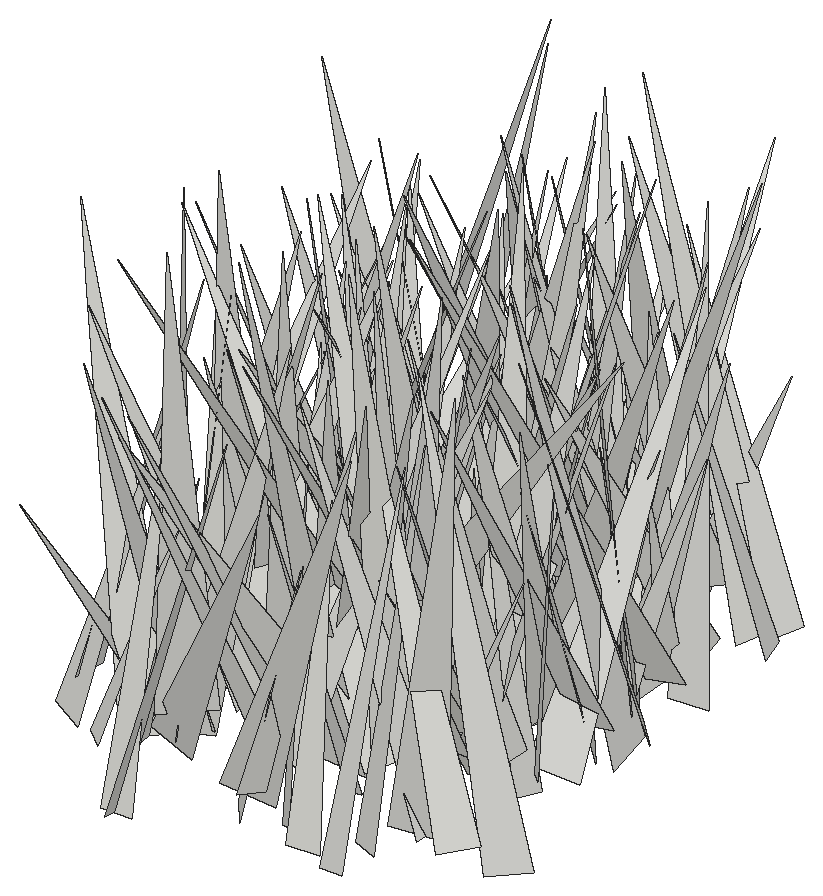
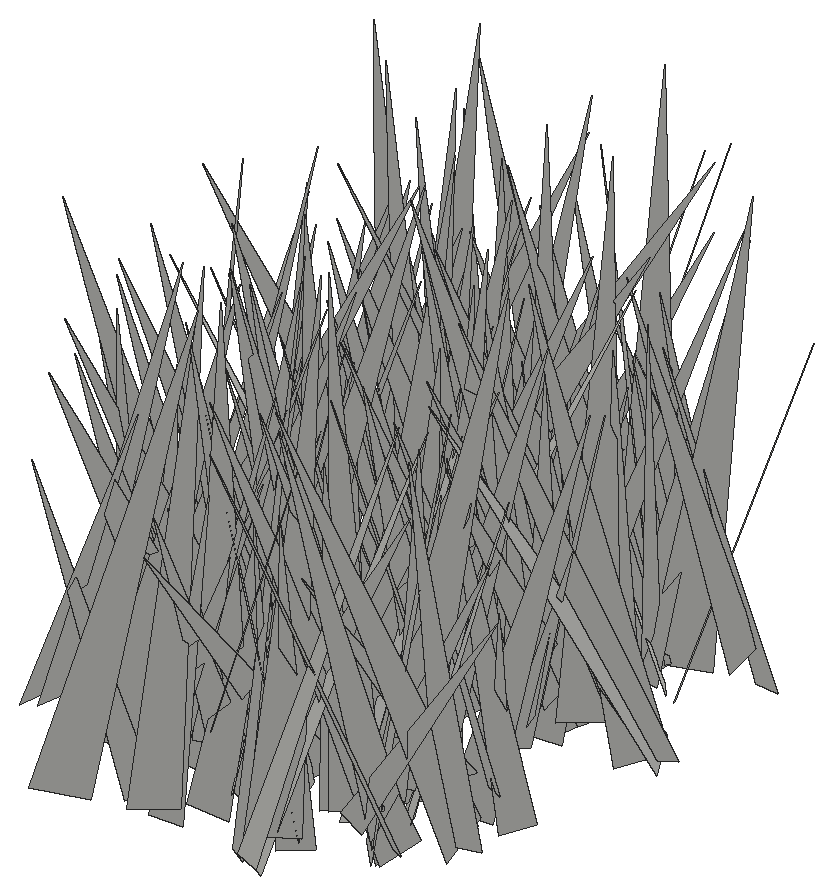
# SketchUp Ruby script. Lengths in inches.
U = 1.inch
M = Sketchup.active_model
def pt(a) = Geom::Point3d.new(a.map { |v| v * U })
def face(e, loops, mat)
  f = e.add_face(loops[0].map { |a| pt(a) })
  loops[1..].each { |l| e.add_face(l.map { |a| pt(a) }).erase! }
  f.material = f.back_material = mat if mat
  f
end
# faces: each face lists its corners as indices into pts; further lists are holes
def faces(e, pts, list, mat = nil) = list.each { |f| face(e, (f[0].is_a?(Array) ? f : [f]).map { |l| l.map { |i| pts[i] } }, mat) }
# xy, xz, yz: faces in a plane at the given z, y or x. An outline is a flat list of corners, or four numbers for a rectangle; further outlines are holes
def ring(l) = l.size == 4 ? [[l[0], l[1]], [l[2], l[1]], [l[2], l[3]], [l[0], l[3]]] : l.each_slice(2).to_a
def flat(e, list, mat, &to3) = list.each { |f| face(e, (f[0].is_a?(Array) ? f : [f]).map { |l| ring(l).map { |u, v| to3.(u, v) } }, mat) }
def xy(e, z, list, mat = nil) = flat(e, list, mat) { |x, y| [x, y, z] }
def xz(e, y, list, mat = nil) = flat(e, list, mat) { |x, z| [x, y, z] }
def yz(e, x, list, mat = nil) = flat(e, list, mat) { |y, z| [x, y, z] }
def lines(e, pts, list) = list.each { |a, b| e.add_line(pt(pts[a]), pt(pts[b])) }
# prism: a flat outline (further loops are holes) pulled along v
def prism(e, loops, v, mat = nil)
  f = face(e, loops, mat); d = Geom::Vector3d.new(v.map { |x| x * U })
  f.pushpull(f.normal.samedirection?(d) ? d.length : -d.length)
end
def box(e, o, s, mat = nil) = prism(e, [[o, [o[0] + s[0], o[1], o[2]], [o[0] + s[0], o[1] + s[1], o[2]], [o[0], o[1] + s[1], o[2]]]], [0, 0, s[2]], mat)
def at(x, y, z, deg = 0) = Geom::Transformation.translation(pt([x, y, z])) * Geom::Transformation.rotation(ORIGIN, Z_AXIS, deg.degrees)
def axes(o, x, y, z) = Geom::Transformation.new([*x, 0, *y, 0, *z, 0, *pt(o).to_a, 1])
def part(name) = M.definitions.add(name)
# library, detail: a bought-in or finely detailed component or shape, given as its bounding box
def library(name, o, s) = part(name).tap { |d| box(d.entities, o, s) }
def detail(e, o, s) = box(e.add_group.entities, o, s)
def put(e, d, t, mat = nil) = e.add_instance(d, t).tap { |i| i.material = mat if mat }
def group(e, t, mat = nil) = e.add_group.tap { |g| g.transformation = t; g.material = mat if mat }.entities
root = M.entities
c1 = part("fur_instance\#9")
p = [[0.8125,0,1.79],[0.67,-0.02,1.48],[0,-0.11,0],[0,0.11,0]]
faces(c1.entities,p,[[0,1,2,3]])
put(root,c1,axes([141.56,90.83,-28.22],[2.97269,-7.01093,0.81561],[-6.80259,-2.60982,2.35986],[1.88234,1.64042,7.24024]))
put(root,c1,axes([139.31,87.79,-28.22],[5.0446,1.96996,1.21492],[1.59207,-5.06819,1.60732],[-1.6799,1.1124,5.17158]))
put(root,c1,axes([139.39,87.84,-28.22],[0.92539,5.82013,0.73982],[5.78512,-1.02986,0.86568],[-0.97656,-0.58571,5.82931]))
put(root,c1,axes([147.1875,87.4,-27.1],[1.91748,5.33638,0.31642],[5.10909,-1.9283,1.55969],[-1.57297,0.24194,5.4517]))
put(root,c1,axes([141.93,89.99,-28.22],[3.37975,2.64749,1.02841],[2.82915,-3.2791,-0.85611],[-0.25046,-1.31446,4.20701]))
put(root,c1,axes([138.12,91.8125,-28.22],[0.97454,-6.53217,0.4424],[-5.83998,-0.6651,3.04417],[2.95966,0.83851,5.86106]))
put(root,c1,axes([140.95,92.76,-28.22],[-5.93761,-4.29126,0.84113],[-3.95201,5.87307,2.0655],[1.8719,-1.21235,7.02879]))
put(root,c1,axes([144.63,89.375,-28.22],[-0.41482,4.98169,1.32883],[5.15587,0.40286,0.09923],[0.00793,-1.33251,4.99795]))
put(root,c1,axes([137.57,89.15,-27.1],[2.54826,3.20038,0.28055],[3.20908,-2.5526,-0.02947],[-0.15164,-0.23787,4.09087]))
put(root,c1,axes([136.37,93.4,-28.22],[-4.06772,-3.26977,0.32403],[-2.78571,3.7053,2.41936],[1.74246,-1.70943,4.62433]))
put(root,c1,axes([138.67,91.83,-27.1],[5.1556,-5.75467,2.21602],[-5.90961,-5.43588,-0.36737],[-1.76168,1.39363,7.71761]))
put(root,c1,axes([140.66,94.3,-28.22],[-5.78164,-4.6449,0.78576],[-4.06196,5.54542,2.89287],[2.386,-1.8147,6.82889]))
put(root,c1,axes([144.97,91.2,-27.1],[0.7235,3.49331,2.20248],[3.65755,-1.58024,1.30491],[-1.91742,-1.69623,3.32022]))
put(root,c1,axes([142.81,89.42,-27.1],[5.29795,0.17393,1.896],[-0.4687,-5.31448,1.7972],[-1.84537,1.84915,4.98684]))
put(root,c1,axes([141.83,93.98,-27.1],[2.44843,-5.51273,0.60157],[-4.8536,-2.44839,-2.68234],[-2.6823,-0.60174,5.40279]))
put(root,c1,axes([146.49,92.05,-28.22],[2.7668,-7.06079,2.0724],[-7.35623,-2.5972,0.97226],[0.18857,2.28135,7.52095]))
put(root,c1,axes([138.97,91.04,-27.1],[5.52113,3.74347,2.2115],[4.00437,-5.77059,-0.2291],[-1.6939,-1.44011,6.66663]))
put(root,c1,axes([138.02,92.97,-28.22],[-0.27695,-6.43694,1.01641],[-6.49492,0.18954,-0.56932],[-0.53231,1.03627,6.4177]))
put(root,c1,axes([137.47,91.25,-28.22],[4.33952,0.70183,1.00017],[0.70812,-4.45199,0.05164],[-0.99573,-0.10739,4.3956]))
put(root,c1,axes([134.91,91.28,-28.22],[2.00403,4.77087,1.2081],[4.88814,-1.77806,-1.08691],[0.57161,-1.52123,5.05925]))
put(root,c1,axes([149.17,90.4375,-27.1],[-2.13966,5.92839,0.3544],[5.56639,1.87053,2.31645],[-2.07043,-1.09766,5.86157]))
put(root,c1,axes([145.89,90.5,-28.22],[2.59525,5.12132,1.23508],[5.09738,-2.78884,0.85303],[-1.33041,-0.69505,5.67763]))
put(root,c1,axes([143.43,90.13,-28.22],[2.74983,3.97442,1.3241],[3.39736,-3.04242,2.07665],[-2.45097,0.24187,4.36407]))
put(root,c1,axes([146.74,92.51,-28.22],[-6.53044,0.59698,0.86107],[0.69842,6.53195,0.76827],[0.78105,-0.84949,6.51251]))
put(root,c1,axes([137.46,91.81,-28.22],[-4.55755,6.1935,2.40469],[6.62517,4.45559,1.08074],[0.49905,-2.58872,7.61332]))
put(root,c1,axes([139.53,93.66,-27.1],[-6.5147,0.26004,1.16019],[0.55336,6.38259,1.67669],[1.05235,-1.74639,6.3006]))
put(root,c1,axes([142.71,93.65,-28.22],[-1.51779,-7.89387,2.17922],[-8.18213,1.37007,-0.73587],[-0.33897,2.275,8.00471]))
put(root,c1,axes([144.74,93.67,-27.1],[4.88048,-6.02987,2.56967],[-6.14977,-5.32095,-0.80587],[-2.26779,1.4525,7.7155]))
put(root,c1,axes([138.14,92.54,-28.22],[4.89354,-4.52263,1.72188],[-4.82903,-4.72322,1.31813],[-0.31551,2.14541,6.53173]))
put(root,c1,axes([146.12,95.57,-28.22],[-1.51333,-7.7582,0.0595],[-7.60064,1.47034,-1.59746],[-1.5568,0.36304,7.74132]))
put(root,c1,axes([149.81,91.84,-28.22],[-2.07893,6.71015,1.41675],[6.64432,1.60395,2.15305],[-1.69892,-1.93817,6.68674]))
put(root,c1,axes([141.61,95.13,-28.22],[6.8807,-3.2851,0.24825],[-3.20439,-6.80705,-1.26238],[-0.76512,-1.03432,7.51946]))
put(root,c1,axes([144.38,95.27,-27.1],[-2.23996,-8.03771,0.28468],[-7.44594,1.96073,-3.22749],[-3.04036,1.11981,7.69451]))
put(root,c1,axes([135.1,92.02,-27.1],[6.05583,0.88682,1.38397],[0.67013,-6.15634,1.01257],[-1.50092,0.82941,6.03608]))
put(root,c1,axes([137.77,92.81,-28.22],[7.69259,-0.4984,1.40276],[-0.64413,-7.77059,0.77146],[-1.3421,0.87272,7.67002]))
put(root,c1,axes([136.98,93.04,-28.22],[2.99336,2.37967,0.42143],[2.41657,-2.95437,-0.48225],[-0.02533,-0.63994,3.79348]))
put(root,c1,axes([140.91,95.33,-28.22],[5.34448,-4.72432,0.68412],[-4.69665,-5.3877,-0.51471],[-0.85369,0.0645,7.11462]))
put(root,c1,axes([144.4375,94.22,-27.1],[0.04247,-7.07988,2.41623],[-7.48051,-0.06275,-0.05238],[-0.06984,2.41579,7.07981]))
put(root,c1,axes([146.44,95.66,-28.22],[-3.08937,-5.14938,0.76665],[-5.09175,3.1744,0.80332],[1.08532,0.23487,5.95105]))
put(root,c1,axes([139.78,94.88,-27.1],[6.66168,-2.88093,2.18206],[-2.80757,-7.00677,-0.67958],[-2.27567,0.211,7.22605]))
put(root,c1,axes([141.04,96.34,-28.22],[-0.1774,-7.7519,1.13116],[-7.17611,0.61466,3.08685],[3.14245,0.96602,7.113]))
put(root,c1,axes([145.93,94.64,-27.1],[-2.3451,-4.39084,0.71964],[-4.31416,2.04482,-1.58228],[-1.08875,1.35503,4.71968]))
put(root,c1,axes([141.49,95.28,-28.22],[-2.67742,-5.68655,1.10676],[-5.79247,2.6077,-0.61446],[-0.09527,1.2623,6.25523]))
put(root,c1,axes([144.76,93.16,-27.1],[-4.02573,7.19257,0.41274],[6.48293,3.4104,3.80141],[-3.14246,-2.17854,7.31361]))
put(root,c1,axes([142.47,91.4375,-27.1],[2.76635,7.35948,0.05567],[7.35952,-2.76581,-0.07342],[0.04914,-0.07794,7.86188]))
put(root,c1,axes([143.23,95.49,-27.1],[0.67729,-7.55263,2.0847],[-7.70125,-0.25666,1.57216],[1.44182,2.17688,7.41817]))
put(root,c1,axes([144.15,96.57,-27.1],[0.26999,-5.16111,0.17986],[-5.16087,-0.27616,-0.17741],[-0.18667,0.17024,5.16512]))
put(root,c1,axes([137.7,92.75,-27.1],[-6.50203,-1.48304,1.94789],[-2.15091,6.10063,-2.53495],[1.1693,2.97539,6.16846]))
put(root,c1,axes([138.15,93.47,-27.1],[0.38602,5.6901,1.15392],[5.67114,-0.61727,1.14668],[-1.24374,-1.04858,5.58671]))
put(root,c1,axes([137.91,96.17,-27.1],[3.24769,-2.54753,0.32293],[-2.51539,-3.26077,-0.4265],[-0.51676,-0.13836,4.10555]))
put(root,c1,axes([141.08,94.61,-28.22],[3.36914,-5.54095,2.01408],[-5.73384,-2.5398,2.60427],[1.37175,2.99283,5.93894]))
put(root,c1,axes([144.87,94.9,-28.22],[2.4928,2.63766,0.46244],[2.65596,-2.35455,-0.88721],[0.34203,-0.94022,3.51911]))
put(root,c1,axes([141.75,95.875,-28.22],[0.54062,-3.9189,1.26852],[-4.01221,-0.79056,-0.73238],[-0.93225,1.12979,3.88763]))
put(root,c1,axes([138.87,94.27,-27.1],[-2.71022,2.78687,0.60598],[2.7235,2.77712,-0.59105],[0.8464,-0.01233,3.84222]))
put(root,c1,axes([147.76,98.07,-27.1],[0.04578,-6.29285,0.19538],[-6.21134,-0.07706,-1.02644],[-1.02831,0.18529,6.20874]))
put(root,c1,axes([136.24,97.27,-27.1],[5.79688,-5.3049,1.7816],[-5.31494,-6.02201,-0.63769],[-1.75142,0.71643,7.83193]))
put(root,c1,axes([137.72,95.67,-28.22],[-2.23187,2.81976,1.51549],[3.01775,2.4697,-0.15093],[1.06816,-1.08561,3.59298]))
put(root,c1,axes([148.3,94.92,-27.1],[2.54415,2.86578,1.34064],[2.68524,-2.86561,1.02977],[-1.67317,-0.2414,3.6912]))
put(root,c1,axes([143.33,95.45,-28.22],[-4.16616,6.68617,2.08588],[7.00105,3.90518,1.46546],[-0.20279,-2.54114,7.74043]))
put(root,c1,axes([147.15,95.55,-27.1],[-5.93557,-1.05009,0.32847],[-1.08922,5.86272,-0.94003],[0.15548,0.98355,5.95399]))
put(root,c1,axes([146.39,97.78,-27.1],[5.5268,-1.95543,1.04999],[-1.67194,-5.52102,-1.48142],[-1.45972,-1.07995,5.67227]))
put(root,c1,axes([137.89,97.21,-28.22],[1.56838,-4.91392,1.31708],[-4.91027,-1.82266,-0.95305],[-1.33063,0.93404,5.06933]))
put(root,c1,axes([137.53,94.9375,-27.1],[-2.26569,5.88907,2.62757],[5.5866,3.18358,-2.31806],[3.22106,-1.37923,5.86866]))
put(root,c1,axes([141.05,98.54,-28.22],[3.47226,-5.91321,0.27335],[-5.89868,-3.48291,-0.41506],[-0.49636,0.02495,6.84473]))
put(root,c1,axes([142.7,96,-28.22],[-3.67972,-3.6806,3.42599],[-4.33109,4.47676,0.15761],[2.55458,2.28831,5.20214]))
put(root,c1,axes([141.54,97.14,-27.1],[-5.94217,-4.1756,0.21971],[-4.13273,5.80684,-1.41225],[-0.63601,1.27993,7.12394]))
put(root,c1,axes([142.625,95.25,-27.1],[-6.42625,-2.81034,1.42452],[-3.14557,5.90814,-2.53441],[0.18076,2.90169,6.53999]))
put(root,c1,axes([135.07,96.42,-28.22],[5.70203,-3.94241,1.833],[-4.2894,-5.59456,1.31056],[-0.70959,2.13867,6.80721]))
put(root,c1,axes([140.96,100.68,-28.22],[4.10096,-6.21113,0.1393],[-5.64172,-3.79303,-3.03306],[-2.60165,-1.56533,6.79681]))
put(root,c1,axes([140.15,96.67,-28.22],[5.80573,-6.03364,0.3689],[-5.4436,-4.99608,3.95649],[2.62833,2.98023,7.37953]))
put(root,c1,axes([147.27,98.74,-28.22],[-3.59225,-3.71334,1.0598],[-3.39845,3.72735,1.54069],[1.83374,-0.36648,4.93148]))
put(root,c1,axes([147.48,95.5625,-28.22],[-5.65883,0.17912,0.29432],[0.09895,5.4838,-1.43499],[0.33003,1.4272,5.47679]))
put(root,c1,axes([138.19,96.77,-27.1],[-3.99726,2.72851,1.81883],[2.89094,4.28575,-0.07581],[1.5477,-0.9584,4.83912]))
put(root,c1,axes([142.34,98.67,-28.22],[6.98287,-2.99298,2.96369],[-2.61118,-7.57832,-1.50091],[-3.30502,-0.33623,7.44753]))
put(root,c1,axes([145.37,98.99,-28.22],[3.60817,-5.34608,1.25489],[-5.24687,-3.79935,-1.09972],[-1.62036,0.39817,6.35531]))
put(root,c1,axes([138.09,97.02,-27.1],[3.39124,-4.48702,2.29298],[-4.9912,-3.37077,0.78574],[-0.69206,2.32297,5.56924]))
put(root,c1,axes([145.99,95.44,-27.1],[3.94824,4.29759,0.4959],[4.2386,-3.97723,0.72087],[-0.86569,0.12707,5.79122]))
put(root,c1,axes([141.38,96.79,-27.1],[-0.70822,-5.57958,3.0516],[-6.3293,0.31925,-0.88519],[-0.61961,3.1164,5.55425]))
put(root,c1,axes([149.0625,98.73,-27.1],[-4.24041,-4.62675,0.86788],[-4.65391,4.29598,0.16351],[0.70788,0.52807,6.27385]))
put(root,c1,axes([138.03,95.74,-27.1],[7.54644,-1.30772,2.23251],[-1.88035,-7.50036,1.96263],[-1.77721,2.38276,7.40318]))
put(root,c1,axes([143.09,96,-27.1],[-5.60196,1.71083,0.59088],[1.59688,5.57635,-1.00614],[0.85208,0.79713,5.77032]))
put(root,c1,axes([140.47,96.3,-27.1],[0.3651,6.79595,1.75212],[7.01816,-0.34958,-0.10649],[0.01583,-1.75528,6.80491]))
put(root,c1,axes([141.18,97.09,-27.1],[4.31663,-3.25233,1.38409],[-3.53279,-4.03972,1.52536],[-0.11299,2.05661,5.185]))
put(root,c1,axes([137.58,97.92,-27.1],[-4.67685,-1.64881,1.07356],[-1.71505,4.77313,-0.14071],[0.96421,0.49258,4.95698]))
put(root,c1,axes([140.96,97.62,-27.1],[-6.02179,2.8816,2.13168],[3.11245,6.27078,0.31555],[1.77772,-1.21792,6.66828]))
put(root,c1,axes([138.78,97.41,-28.22],[4.6922,-0.3007,0.23761],[-0.32477,-4.66947,0.50417],[-0.20347,0.51889,4.67471]))
put(root,c1,axes([140.3125,98.25,-27.1],[5.34451,-3.5502,0.35957],[-3.55754,-5.25077,1.03462],[0.27778,1.05952,6.33224]))
put(root,c1,axes([143.46,98.27,-27.1],[3.51099,-0.42801,1.09439],[-0.295,-3.65871,-0.48452],[-1.13748,-0.37227,3.50364]))
put(root,c1,axes([148.21,99.06,-28.22],[-7.391,-1.41623,2.02124],[-1.14457,7.62073,1.15434],[2.18657,-0.79801,7.4364]))
put(root,c1,axes([136.15,96.97,-27.1],[3.23121,-4.00646,1.7311],[-4.24322,-2.37965,2.41277],[1.02152,2.78831,4.54653]))
put(root,c1,axes([138.74,97.01,-27.1],[-2.41477,3.3901,0.55663],[3.41153,2.44646,-0.10002],[0.40504,-0.3947,4.161]))
put(root,c1,axes([138.11,98.02,-28.22],[-3.21224,1.96871,0.46482],[2.01704,3.18335,0.45637],[0.15311,-0.63315,3.7398]))
put(root,c1,axes([140.5,98.74,-28.22],[-2.84095,-2.72325,0.75235],[-2.80656,2.8428,-0.30791],[0.32453,0.74533,3.9233]))
put(root,c1,axes([134.83,96.24,-28.22],[-0.55252,7.61083,1.2014],[7.43516,0.84266,-1.91879],[2.02152,-1.01911,7.38568]))
put(root,c1,axes([145.11,96.95,-28.22],[5.43285,-3.6045,3.64876],[-4.74936,-5.54221,1.59663],[-1.93634,3.48041,6.32132]))
put(root,c1,axes([134.83,95.89,-28.22],[6.18332,3.30926,0.01495],[3.17233,-5.93637,1.96995],[-0.9422,1.73008,6.73082]))
put(root,c1,axes([147.73,101.24,-27.1],[-1.57704,-7.74459,0.50786],[-7.45096,1.36569,-2.31124],[-2.17253,0.93802,7.55804]))
put(root,c1,axes([138.4,100.46,-28.22],[-0.43336,-3.79274,0.22877],[-3.61563,0.48241,1.14868],[1.16807,0.08612,3.64049]))
put(root,c1,axes([137.57,95.99,-28.22],[-4.59878,4.14257,0.47856],[3.69105,4.37512,-2.40275],[1.94062,1.49539,5.70408]))
put(root,c1,axes([144.63,97.96,-27.1],[-6.2785,3.87073,1.88034],[3.7817,6.55006,-0.85632],[2.05354,-0.22787,7.32591]))
put(root,c1,axes([139.14,103.98,-28.22],[-5.00279,-6.48805,0.18943],[-5.66686,4.48249,3.86684],[3.16501,-2.22958,7.22289]))
put(root,c1,axes([147.68,99.69,-27.1],[-5.07554,-4.81191,2.50581],[-5.17107,5.32884,-0.24106],[1.64121,1.90882,6.98981]))
put(root,c1,axes([147.29,96.91,-28.22],[-1.59566,7.05244,0.57454],[6.94745,1.67322,-1.24356],[1.34162,-0.27674,7.12297]))
put(root,c1,axes([138.97,100.48,-27.1],[1.01091,-5.94061,2.30759],[-6.04054,-1.63799,-1.57056],[-2.03168,1.91413,5.81775]))
put(root,c1,axes([144.35,98.95,-27.1],[4.3038,1.80689,1.01933],[1.67441,-4.41138,0.75005],[-1.22483,0.31842,4.60705]))
put(root,c1,axes([144.78,96.58,-27.1],[5.37795,5.75,0.47067],[5.40496,-5.24661,2.33794],[-2.01755,1.27162,7.51791]))
put(root,c1,axes([136.77,101.7,-28.22],[2.07945,-5.56592,1.40736],[-5.43571,-2.39045,-1.42237],[-1.84751,0.76846,5.76892]))
put(root,c1,axes([140.52,101.72,-28.22],[2.77166,-6.45652,0.14972],[-5.9267,-2.47813,2.8503],[2.56578,1.25036,6.42219]))
put(root,c1,axes([145.32,100.43,-27.1],[4.26673,-0.51352,0.23406],[-0.5171,-4.27238,0.05285],[-0.22604,0.08052,4.29719]))
put(root,c1,axes([137.9,98.77,-27.1],[6.18202,1.83786,0.77531],[1.68935,-6.16651,1.14736],[-1.06062,0.8903,6.34654]))
put(root,c1,axes([146.68,101.38,-28.22],[3.60771,1.96245,2.32029],[2.67745,-3.75626,-0.98607],[-1.43745,-2.07119,3.98679]))
put(root,c1,axes([142.08,100.49,-28.22],[-6.66331,2.16551,0.21128],[2.17487,6.60915,0.85019],[-0.06344,-0.87375,6.95459]))
put(root,c1,axes([143.98,103.41,-27.1],[-0.13701,-6.93499,0.01519],[-6.899,0.13785,0.70555],[0.70571,0.00117,6.90036]))
put(root,c1,axes([138.12,102.54,-28.22],[-3.04266,-3.74721,0.50143],[-3.60797,3.07034,1.05183],[1.12942,-0.28668,4.71094]))
put(root,c1,axes([142.22,104.12,-27.1],[1.01288,-8.11783,0.06805],[-8.08119,-1.01477,-0.77093],[-0.77341,-0.02823,8.14437]))
put(root,c1,axes([143.96,103.61,-28.22],[-3.9218,-4.42687,0.35438],[-4.07666,3.77609,2.05553],[1.7617,-1.11678,5.54549]))
put(root,c1,axes([141.82,101.53,-27.1],[5.79925,-1.98106,0.58125],[-1.98372,-5.82701,-0.06806],[-0.57211,0.1232,6.12791]))
put(root,c1,axes([143.58,101.29,-28.22],[6.48225,-3.39085,0.68777],[-3.4557,-6.41712,0.9323],[-0.17042,1.14593,7.25591]))
put(root,c1,axes([137.03,99.99,-28.22],[-0.19051,3.61425,0.52762],[3.57644,0.0773,0.76192],[-0.74175,-0.55561,3.53816]))
put(root,c1,axes([139.27,99.91,-27.1],[4.10356,-2.98524,2.70877],[-3.77942,-4.1935,1.10399],[-1.40181,2.56732,4.95298]))
put(root,c1,axes([135.28,101.46,-28.22],[4.86131,-2.02952,0.59697],[-2.06386,-4.87843,0.22145],[-0.46454,0.43544,5.26329]))
put(root,c1,axes([142.24,98.49,-28.22],[3.83849,6.3713,1.10198],[6.13828,-3.99344,1.70758],[-2.03209,-0.02789,7.23959]))
put(root,c1,axes([146.2,101.13,-28.22],[1.01992,4.1189,1.46608],[4.23417,-0.55549,-1.38501],[1.0893,-1.69737,4.0109]))
put(root,c1,axes([146.45,104.46,-28.22],[-6.04066,-0.63869,2.51357],[0.73038,5.69455,3.20222],[2.48847,-3.22176,5.16172]))
put(root,c1,axes([139.01,101.02,-27.1],[-4.50468,1.1443,0.55643],[1.12699,4.53841,-0.20945],[0.5907,0.0676,4.64302]))
put(root,c1,axes([145.96,100.49,-27.1],[6.16496,0.12051,1.82007],[-0.27856,-6.27765,1.3592],[-1.80266,1.38221,6.01447]))
put(root,c1,axes([144.43,102.32,-28.22],[-2.07432,-2.92088,0.84042],[-3.01146,2.11274,-0.09003],[0.41107,0.73854,3.58137]))
put(root,c1,axes([146.63,102.87,-28.22],[1.50784,-3.41822,0.5063],[-3.4457,-1.52893,-0.06057],[-0.26023,0.4385,3.73552]))
put(root,c1,axes([145.11,104.15,-28.22],[1.95168,-6.84621,1.26966],[-6.52036,-2.2596,-2.16121],[-2.44285,0.56154,6.78298]))
put(root,c1,axes([135.84,101.77,-27.1],[2.6257,3.60497,0.95618],[3.72031,-2.44904,-0.98281],[0.26337,-1.34567,4.35019]))
put(root,c1,axes([145.86,102.2,-28.22],[4.85202,-3.37562,1.03104],[-3.52041,-4.75453,1.00059],[-0.25408,1.41409,5.82544]))
put(root,c1,axes([136.61,101.75,-28.22],[4.20289,4.66758,0.96744],[4.74909,-3.98911,-1.38552],[0.41036,-1.63927,6.12625]))
put(root,c1,axes([138.06,103.125,-27.1],[2.50523,-6.92108,2.84903],[-7.08461,-3.16179,-1.45116],[-2.41383,2.09672,7.21607]))
put(root,c1,axes([143.01,100.62,-27.1],[-6.71814,2.72987,2.53139],[2.23652,7.13443,-1.75826],[2.97626,0.8008,7.03521]))
put(root,c1,axes([146.48,102.08,-28.22],[-7.94923,-1.56442,0.5472],[-1.62855,7.87073,-1.15603],[0.30767,1.24144,8.0188]))
put(root,c1,axes([137.81,103.89,-27.1],[2.72704,-3.27265,0.76108],[-3.17295,-2.83078,-0.80329],[-1.10537,0.05182,4.1835]))
put(root,c1,axes([141.07,103.1,-28.22],[3.2608,1.42212,0.87051],[1.60342,-3.19897,-0.78016],[-0.45742,-1.07574,3.47082]))
put(root,c1,axes([138.38,102,-28.22],[-4.60516,3.74944,1.60687],[3.84875,4.79672,-0.16237],[1.35183,-0.88372,5.93628]))
put(root,c1,axes([142.1,101.54,-28.22],[4.26964,0.47793,1.18834],[0.14194,-4.28676,1.21405],[-1.27296,1.12502,4.1212]))
put(root,c1,axes([137.48,103.6,-28.22],[-4.16981,-3.31895,0.85743],[-3.36405,4.22145,-0.01946],[0.65859,0.54939,5.32938]))
put(root,c1,axes([140.31,101.87,-28.22],[7.3545,-2.24014,2.18394],[-2.66673,-7.40612,1.38362],[-1.63595,2.00191,7.56257]))
put(root,c1,axes([138.07,104.9,-27.1],[2.36593,-6.95857,0.28973],[-6.83072,-2.25873,1.53056],[1.359,0.76137,7.18865]))
put(root,c1,axes([145.96,102.71,-28.22],[2.31719,-2.3997,1.71249],[-2.74416,-2.55172,0.13746],[-1.07739,1.33819,3.33302]))
put(root,c1,axes([146.21,103.12,-27.1],[-1.45922,4.42701,2.15741],[4.90506,1.50733,0.22462],[0.43952,-2.12407,4.65589]))
put(root,c1,axes([144.89,102.05,-27.1],[7.47756,-1.51643,1.55812],[-1.8154,-7.42558,1.48539],[-1.19651,1.78955,7.48379]))
put(root,c1,axes([138.95,103.43,-28.22],[-3.88127,2.88585,0.74535],[2.95869,3.58243,1.53633],[-0.36036,-1.66913,4.58608]))
put(root,c1,axes([144.93,102.91,-28.22],[-3.14224,2.77876,1.0294],[2.91205,3.17344,0.32264],[0.54877,-0.92877,4.18224]))
put(root,c1,axes([140.47,100.51,-28.22],[0.11708,7.08162,0.20269],[7.08451,-0.11681,-0.01106],[0.00771,-0.20285,7.08258]))
put(root,c1,axes([144.78,101.15,-27.1],[-3.66435,5.27166,1.90181],[4.6134,4.12758,-2.55233],[3.18179,0.08644,5.89097]))
put(root,c1,axes([144.33,105.21,-27.1],[1.81992,-3.21241,0.00061],[-3.09433,-1.75321,-0.99152],[-0.86298,-0.48823,3.55649]))
put(root,c1,axes([143.84,101.9,-27.1],[-6.0255,1.4926,2.28597],[0.94971,6.33899,-1.63567],[2.5596,1.16168,5.98825]))
put(root,c1,axes([147.74,102.21,-28.22],[0.42916,7.00561,1.64499],[7.11073,-0.66598,0.98114],[-1.10544,-1.56418,6.94983]))
put(root,c1,axes([135.86,103.19,-28.22],[-0.55684,5.82392,2.02647],[6.12632,0.75415,-0.48394],[0.70204,-1.96161,5.83043]))
put(root,c1,axes([136.97,100.99,-28.22],[-2.44099,4.81015,0.04297],[4.37742,2.2412,-2.21652],[1.99437,0.96814,4.91762]))
put(root,c1,axes([148.91,104.38,-27.1],[-4.66141,-1.64687,0.68606],[-1.65466,4.70851,0.06011],[0.66704,0.1713,4.94341]))
put(root,c1,axes([145.32,106.09,-27.1],[2.99002,-5.93259,1.12286],[-5.76165,-3.17812,-1.449],[-1.8055,0.31717,6.48354]))
put(root,c1,axes([142.36,105.88,-28.22],[-0.18064,-6.52008,0.8881],[-6.57997,0.17015,-0.08916],[-0.06535,0.89016,6.52198]))
put(root,c1,axes([137.61,104.93,-28.22],[4.20893,3.73459,3.7879],[4.59902,-4.98198,-0.19834],[-2.67289,-2.69131,5.62342]))
put(root,c1,axes([141.33,106.13,-27.1],[-4.0085,-3.44331,0.94309],[-3.06456,4.04605,1.74695],[1.83147,-0.76613,4.98725]))
put(root,c1,axes([139.67,103.45,-28.22],[3.60386,-3.42869,2.87422],[-4.08632,-4.02533,0.32181],[-1.82182,2.24626,4.96388]))
put(root,c1,axes([144.27,103.08,-27.1],[-5.43034,-1.89464,0.64767],[-1.9986,5.01546,-2.08529],[-0.12137,2.18018,5.36002]))
put(root,c1,axes([138.91,107.42,-27.1],[6.44625,-4.17663,0.34492],[-3.99481,-6.31514,-1.81045],[-1.26676,-1.33867,7.46462]))
put(root,c1,axes([137.73,105.53,-27.1],[-0.38653,-3.78857,0.47263],[-3.40937,0.1287,-1.7566],[-1.71837,0.59684,3.37891]))
put(root,c1,axes([140.28,107.2,-28.22],[-4.91582,-6.36103,2.07601],[-5.8042,5.33544,2.60426],[3.32923,-0.09063,7.60565]))
put(root,c1,axes([139.66,105.37,-28.22],[5.79589,4.16761,1.50359],[4.42839,-5.37215,-2.17978],[0.13803,-2.64446,6.79779]))
put(root,c1,axes([139.52,107.45,-28.22],[-3.98509,-5.15803,0.00595],[-5.07141,3.91953,1.18509],[0.94137,-0.71992,6.40951]))
put(root,c1,axes([141.99,104.78,-28.22],[-1.81659,5.58818,1.87966],[5.39696,0.78429,2.88421],[-2.37355,-2.49359,5.11948]))
put(root,c1,axes([141.11,104.68,-28.22],[1.95895,3.98258,1.69888],[4.26762,-2.09086,-0.01944],[-0.73116,-1.53362,4.43825]))
put(root,c1,axes([136.92,104.4375,-28.22],[6.85637,-0.90607,0.05149],[-0.90407,-6.7849,0.99057],[0.07926,0.98874,6.84468]))
put(root,c1,axes([143.08,104.4,-27.1],[-2.11891,6.73628,2.3501],[7.12334,2.13432,0.30482],[0.39806,-2.33612,7.05509]))
put(root,c1,axes([143.9,105.1875,-27.1],[-3.99562,-4.42007,1.47298],[-4.65768,3.83659,-1.12173],[0.11293,1.84803,5.85182]))
put(root,c1,axes([142.59,104.47,-27.1],[-0.05946,3.80591,1.08242],[3.88392,0.26301,-0.71143],[0.75616,-1.05166,3.7393]))
put(root,c1,axes([145.18,103.2,-27.1],[5.43487,-1.88004,3.06705],[-2.9758,-5.47185,1.91904],[-2.02138,3.00059,5.42123]))
put(root,c1,axes([148.13,104.85,-27.1],[-8.02945,1.44749,0.94959],[1.4539,8.08421,-0.0293],[0.93976,-0.13944,8.15883]))
put(root,c1,axes([145.75,101.89,-27.1],[-4.59589,5.78444,0.11594],[5.4804,4.40003,-2.28044],[1.8543,1.33244,7.02721]))
put(root,c1,axes([141.33,102.32,-28.22],[-3.68567,4.23937,0.30212],[3.60627,3.33103,-2.74713],[2.24908,1.60613,4.89997]))
put(root,c1,axes([143.55,106.85,-27.1],[-0.33962,-4.53633,0.58104],[-4.49375,0.22275,-0.88758],[-0.84975,0.63509,4.46159]))
put(root,c1,axes([139.24,106.02,-28.22],[-2.45808,3.26284,2.53045],[3.74921,2.99751,-0.22312],[1.72995,-1.86016,4.07903]))
put(root,c1,axes([136.04,102.81,-28.22],[7.79418,1.63756,2.08164],[0.8535,-7.67768,2.8441],[-2.50726,2.47704,7.43922]))
put(root,c1,axes([142.36,108.1875,-27.1],[6.58115,-3.41587,1.26301],[-3.10443,-6.62563,-1.74311],[-1.90417,-1.00387,7.20703]))
put(root,c1,axes([148.61,105.33,-27.1],[-5.80532,1.01557,0.17125],[1.00882,5.80466,-0.22508],[0.20737,0.19232,5.88918]))
put(root,c1,axes([142.79,103.99,-28.22],[-2.87102,4.68172,0.40163],[4.57171,2.89185,-1.02921],[1.08596,0.20316,5.39463]))
put(root,c1,axes([144.24,106.36,-28.22],[1.52627,-4.48364,1.33128],[-4.39877,-0.90019,2.01128],[1.58937,1.81423,4.28804]))
put(root,c1,axes([138.62,108.88,-27.1],[-3.25593,-5.45811,0.05054],[-5.36708,3.21208,1.12765],[0.99394,-0.53501,6.25464]))
put(root,c1,axes([142.96,106.93,-28.22],[0.46643,-4.66615,1.44002],[-4.86096,-0.58186,-0.31092],[-0.46655,1.39737,4.67909]))
put(root,c1,axes([137.36,104.22,-28.22],[-6.79191,0.51616,3.38033],[-0.49773,7.28774,-2.11287],[3.3831,2.10844,6.47551]))
put(root,c1,axes([146.08,107.56,-28.22],[4.0303,-5.81988,3.12764],[-5.66664,-4.92868,-1.86917],[-3.39741,1.31665,6.82792]))
put(root,c1,axes([135.79,106,-27.1],[4.10268,4.53992,0.30052],[4.35228,-3.79801,-2.04106],[1.3262,-1.58032,5.76861]))
